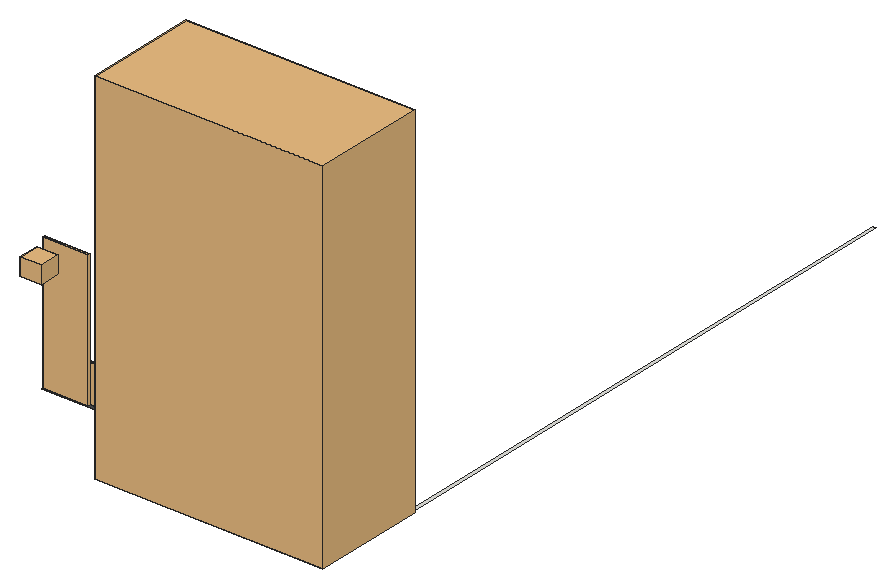
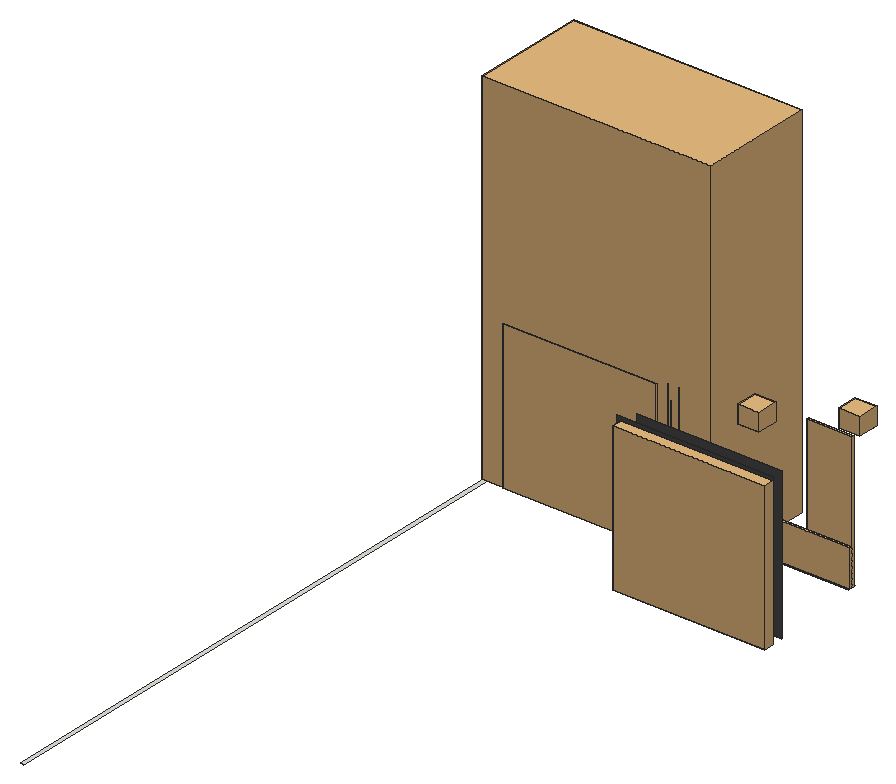
# SketchUp Ruby script. Lengths in inches.
U = 1.inch
M = Sketchup.active_model
def pt(a) = Geom::Point3d.new(a.map { |v| v * U })
def face(e, loops, mat)
  f = e.add_face(loops[0].map { |a| pt(a) })
  loops[1..].each { |l| e.add_face(l.map { |a| pt(a) }).erase! }
  f.material = f.back_material = mat if mat
  f
end
# faces: each face lists its corners as indices into pts; further lists are holes
def faces(e, pts, list, mat = nil) = list.each { |f| face(e, (f[0].is_a?(Array) ? f : [f]).map { |l| l.map { |i| pts[i] } }, mat) }
# xy, xz, yz: faces in a plane at the given z, y or x. An outline is a flat list of corners, or four numbers for a rectangle; further outlines are holes
def ring(l) = l.size == 4 ? [[l[0], l[1]], [l[2], l[1]], [l[2], l[3]], [l[0], l[3]]] : l.each_slice(2).to_a
def flat(e, list, mat, &to3) = list.each { |f| face(e, (f[0].is_a?(Array) ? f : [f]).map { |l| ring(l).map { |u, v| to3.(u, v) } }, mat) }
def xy(e, z, list, mat = nil) = flat(e, list, mat) { |x, y| [x, y, z] }
def xz(e, y, list, mat = nil) = flat(e, list, mat) { |x, z| [x, y, z] }
def yz(e, x, list, mat = nil) = flat(e, list, mat) { |y, z| [x, y, z] }
def lines(e, pts, list) = list.each { |a, b| e.add_line(pt(pts[a]), pt(pts[b])) }
# prism: a flat outline (further loops are holes) pulled along v
def prism(e, loops, v, mat = nil)
  f = face(e, loops, mat); d = Geom::Vector3d.new(v.map { |x| x * U })
  f.pushpull(f.normal.samedirection?(d) ? d.length : -d.length)
end
def box(e, o, s, mat = nil) = prism(e, [[o, [o[0] + s[0], o[1], o[2]], [o[0] + s[0], o[1] + s[1], o[2]], [o[0], o[1] + s[1], o[2]]]], [0, 0, s[2]], mat)
def at(x, y, z, deg = 0) = Geom::Transformation.translation(pt([x, y, z])) * Geom::Transformation.rotation(ORIGIN, Z_AXIS, deg.degrees)
def axes(o, x, y, z) = Geom::Transformation.new([*x, 0, *y, 0, *z, 0, *pt(o).to_a, 1])
def part(name) = M.definitions.add(name)
# library, detail: a bought-in or finely detailed component or shape, given as its bounding box
def library(name, o, s) = part(name).tap { |d| box(d.entities, o, s) }
def detail(e, o, s) = box(e.add_group.entities, o, s)
def put(e, d, t, mat = nil) = e.add_instance(d, t).tap { |i| i.material = mat if mat }
def group(e, t, mat = nil) = e.add_group.tap { |g| g.transformation = t; g.material = mat if mat }.entities
root = M.entities
M.materials.add("1423 AP 8230 BENTONITE").color = [77, 75, 77]
M.materials.add("1427 AP 686 ARMOUR-N").color = [184, 186, 189]
M.materials.add("[Wood Cherry Original]").color = [100, 65, 42]
M.materials.add("[Wood Veneer 01]").color = [99, 65, 43]
c1 = library("Curtains",[0,0,0],[121.73,8.19,117.22])
c2 = library("Group\#13",[-25,-1,0],[182,91,288])
c3 = library("Untitled",[0,0,0],[96,5.09,80])
c4 = library("Group\#19",[0,-2,0],[36,2,114])
c5 = library("Group\#35",[-36,0,0],[116,2,29.75])
c6 = library("2",[-6.43,-6.43,-13.78],[16.84,16.84,13.78])
xy(root,126,[[287,192,290,672]])
xy(root,126,[[151.78,192,151.57,192.01,151.35,192.01,150.91,192.03,150.7,192.05,150.48,192.0625,150.26,192.08,150.05,192.11,149.83,192.13,149.61,192.16,149.4,192.1875,149.18,192.22,148.97,192.26,148.76,192.29,148.54,192.34,148.12,192.42,147.9,192.47,147.69,192.52,147.48,192.58,147.27,192.63,147.0625,192.69,146.85,192.75,146.64,192.82,146.4375,192.88,146.23,192.95,146.03,193.02,145.82,193.09,145.62,193.17,145.41,193.25,145.01,193.41,144.8125,193.5,144.61,193.59,144.41,193.68,144.22,193.77,144.02,193.86,143.83,193.96,143.63,194.0625,143.44,194.16,143.25,194.27,142.875,194.48,142.6875,194.6,142.5,194.71,142.32,194.83,142.14,194.94,141.95,195.0625,141.77,195.1875,141.6,195.3125,141.42,195.4375,141.24,195.57,140.9,195.83,140.73,195.97,140.56,196.1,140.39,196.24,140.23,196.38,140.0625,196.53,139.9,196.67,139.58,196.97,139.43,197.12,139.27,197.27,139.12,197.43,138.97,197.58,138.67,197.9,138.53,198.0625,138.38,198.23,138.24,198.39,138.1,198.56,137.97,198.73,137.83,198.9,137.57,199.24,137.4375,199.42,137.3125,199.6,137.1875,199.77,137.0625,199.95,136.94,200.14,136.83,200.32,136.71,200.5,136.6,200.6875,136.48,200.875,136.27,201.25,136.16,201.44,136.0625,201.63,135.96,201.83,135.86,202.02,135.77,202.22,135.68,202.41,135.59,202.61,135.5,202.8125,135.41,203.01,135.25,203.41,135.17,203.62,135.09,203.82,135.02,204.03,134.95,204.23,134.88,204.4375,134.82,204.64,134.75,204.85,134.69,205.0625,134.63,205.27,134.58,205.48,134.52,205.69,134.47,205.9,134.42,206.12,134.34,206.54,134.29,206.76,134.26,206.97,134.22,207.18,134.1875,207.4,134.16,207.61,134.13,207.83,134.11,208.05,134.08,208.26,134.0625,208.48,134.05,208.7,134.03,208.91,134.01,209.35,134.01,209.57,134,209.78,134,252,128,252,128,261,143,261,143,209.78,143.01,209.67,143.01,209.57,143.02,209.46,143.02,209.35,143.05,209.02,143.07,208.92,143.09,208.7,143.13,208.48,143.15,208.38,143.17,208.27,143.1875,208.16,143.21,208.06,143.24,207.95,143.26,207.85,143.29,207.74,143.32,207.64,143.35,207.53,143.375,207.43,143.41,207.32,143.47,207.12,143.51,207.01,143.55,206.91,143.58,206.81,143.625,206.71,143.66,206.61,143.71,206.51,143.79,206.31,143.84,206.21,143.88,206.11,143.98,205.91,144.03,205.82,144.08,205.72,144.13,205.625,144.1875,205.53,144.24,205.4375,144.3,205.34,144.35,205.25,144.59,204.89,144.66,204.8,144.78,204.62,144.85,204.54,144.92,204.45,144.98,204.36,145.12,204.2,145.19,204.11,145.26,204.03,145.34,203.95,145.48,203.79,145.56,203.71,145.64,203.64,145.71,203.56,145.79,203.48,145.95,203.34,146.03,203.26,146.11,203.19,146.2,203.12,146.36,202.98,146.45,202.92,146.54,202.85,146.62,202.78,146.8,202.66,146.89,202.59,147.25,202.35,147.34,202.3,147.4375,202.24,147.53,202.1875,147.625,202.13,147.72,202.08,147.82,202.03,147.91,201.98,148.11,201.88,148.21,201.84,148.31,201.79,148.51,201.71,148.61,201.66,148.71,201.625,148.81,201.58,148.91,201.55,149.01,201.51,149.12,201.47,149.32,201.41,149.43,201.375,149.53,201.35,149.64,201.32,149.74,201.29,149.85,201.26,149.95,201.24,150.06,201.21,150.16,201.1875,150.27,201.17,150.38,201.15,150.48,201.13,150.7,201.09,150.92,201.07,151.02,201.05,151.35,201.02,151.46,201.02,151.57,201.01,151.67,201.01,151.78,201,170,201,170,192]],"1423 AP 8230 BENTONITE")
xy(root,132,[[18,180,134,186]],"1423 AP 8230 BENTONITE")
xy(root,216,[[56,252,128,261]],"1423 AP 8230 BENTONITE")
xy(root,222,[[170,192,254,201]],"1423 AP 8230 BENTONITE")
xz(root,201,[[151.78,126,151.89,246],[151.89,126,151.89,246,281,246,281,126,254,126,254,222,170,222,170,126]],"1423 AP 8230 BENTONITE")
xz(root,201.01,[[151.57,126,151.67,246]],"1423 AP 8230 BENTONITE")
xz(root,201.02,[[151.35,126,151.46,246]],"1423 AP 8230 BENTONITE")
xz(root,252,[[18,126,56,126,56,216,128,216,128,126,134,126,134,246,18,246]],"1423 AP 8230 BENTONITE")
xz(root,261,[[18,126,18,246,143,246,143,126,128,126,128,216,56,216,56,126]],"1423 AP 8230 BENTONITE")
yz(root,56,[[252,126,261,216]],"1423 AP 8230 BENTONITE")
yz(root,128,[[252,126,261,216]],"1423 AP 8230 BENTONITE")
yz(root,134,[[209.78,126,210,246]],"1423 AP 8230 BENTONITE")
yz(root,134.01,[[209.35,126,209.57,246]],"1423 AP 8230 BENTONITE")
yz(root,143,[[209.78,126,209.89,246]],"1423 AP 8230 BENTONITE")
yz(root,143.01,[[209.57,126,209.67,246]],"1423 AP 8230 BENTONITE")
yz(root,143.02,[[209.35,126,209.46,246]],"1423 AP 8230 BENTONITE")
p = [[151.02,201.05,246],[151.13,201.04,246],[151.13,201.04,126],[151.02,201.05,126],[151.24,201.03,246],[151.24,201.03,126],
  [151.35,201.02,246],[151.35,201.02,126],[151.46,201.02,246],[151.57,201.01,246],[151.57,201.01,126],[151.46,201.02,126],
  [151.67,201.01,246],[151.78,201,246],[151.78,201,126],[151.67,201.01,126],[150.27,201.17,246],[150.38,201.15,246],
  [150.38,201.15,126],[150.27,201.17,126],[150.48,201.13,246],[150.48,201.13,126],[150.59,201.11,246],[150.59,201.11,126],
  [150.7,201.09,246],[150.7,201.09,126],[150.81,201.08,246],[150.81,201.08,126],[150.92,201.07,246],[150.92,201.07,126],
  [149.85,201.26,246],[149.95,201.24,246],[149.95,201.24,126],[149.85,201.26,126],[150.06,201.21,246],[150.06,201.21,126],
  [150.16,201.1875,246],[150.16,201.1875,126],[149.43,201.375,246],[149.53,201.35,246],[149.53,201.35,126],[149.43,201.375,126],
  [149.64,201.32,246],[149.64,201.32,126],[149.74,201.29,246],[149.74,201.29,126],[149.12,201.47,246],[149.22,201.44,246],
  [149.22,201.44,126],[149.12,201.47,126],[149.32,201.41,246],[149.32,201.41,126],[148.81,201.58,246],[148.91,201.55,246],
  [148.91,201.55,126],[148.81,201.58,126],[149.01,201.51,246],[149.01,201.51,126],[148.61,201.66,246],[148.71,201.625,246],
  [148.71,201.625,126],[148.61,201.66,126],[148.31,201.79,246],[148.41,201.75,246],[148.41,201.75,126],[148.31,201.79,126],
  [148.51,201.71,246],[148.51,201.71,126],[148.11,201.88,246],[148.21,201.84,246],[148.21,201.84,126],[148.11,201.88,126],
  [147.91,201.98,246],[148.01,201.93,246],[148.01,201.93,126],[147.91,201.98,126],[147.72,202.08,246],[147.82,202.03,246],
  [147.82,202.03,126],[147.72,202.08,126],[147.53,202.1875,246],[147.625,202.13,246],[147.625,202.13,126],[147.53,202.1875,126],
  [147.34,202.3,246],[147.4375,202.24,246],[147.4375,202.24,126],[147.34,202.3,126],[147.25,202.35,246],[147.25,202.35,126],
  [147.07,202.47,246],[147.16,202.41,246],[147.16,202.41,126],[147.07,202.47,126],[146.89,202.59,246],[146.98,202.53,246],
  [146.98,202.53,126],[146.89,202.59,126],[146.8,202.66,246],[146.8,202.66,126],[146.62,202.78,246],[146.71,202.72,246],
  [146.71,202.72,126],[146.62,202.78,126],[146.45,202.92,246],[146.54,202.85,246],[146.54,202.85,126],[146.45,202.92,126],
  [146.36,202.98,246],[146.36,202.98,126],[146.28,203.05,246],[146.28,203.05,126],[146.11,203.19,246],[146.2,203.12,246],
  [146.2,203.12,126],[146.11,203.19,126],[146.03,203.26,246],[146.03,203.26,126],[145.87,203.41,246],[145.95,203.34,246],
  [145.95,203.34,126],[145.87,203.41,126],[145.79,203.48,246],[145.79,203.48,126],[145.71,203.56,246],[145.71,203.56,126],
  [145.64,203.64,246],[145.64,203.64,126],[145.56,203.71,246],[145.56,203.71,126],[145.48,203.79,246],[145.48,203.79,126],
  [145.41,203.87,246],[145.41,203.87,126],[145.34,203.95,246],[145.34,203.95,126],[145.19,204.11,246],[145.26,204.03,246],
  [145.26,204.03,126],[145.19,204.11,126],[145.12,204.2,246],[145.12,204.2,126],[145.05,204.28,246],[145.05,204.28,126],
  [144.98,204.36,246],[144.98,204.36,126],[144.85,204.54,246],[144.92,204.45,246],[144.92,204.45,126],[144.85,204.54,126],
  [144.78,204.62,246],[144.78,204.62,126],[144.72,204.71,246],[144.72,204.71,126],[144.66,204.8,246],[144.66,204.8,126],
  [144.59,204.89,246],[144.59,204.89,126],[144.53,204.98,246],[144.53,204.98,126],[144.47,205.07,246],[144.47,205.07,126],
  [144.41,205.16,246],[144.41,205.16,126],[144.35,205.25,246],[144.35,205.25,126],[144.24,205.4375,246],[144.3,205.34,246],
  [144.3,205.34,126],[144.24,205.4375,126],[144.1875,205.53,246],[144.1875,205.53,126],[144.13,205.625,246],[144.13,205.625,126],
  [144.08,205.72,246],[144.08,205.72,126],[144.03,205.82,246],[144.03,205.82,126],[143.98,205.91,246],[143.98,205.91,126],
  [143.93,206.01,246],[143.93,206.01,126],[143.88,206.11,246],[143.88,206.11,126],[143.84,206.21,246],[143.84,206.21,126],
  [143.79,206.31,246],[143.79,206.31,126],[143.75,206.41,246],[143.75,206.41,126],[143.71,206.51,246],[143.71,206.51,126],
  [143.66,206.61,246],[143.66,206.61,126],[143.625,206.71,246],[143.625,206.71,126],[143.58,206.81,246],[143.58,206.81,126],
  [143.55,206.91,246],[143.55,206.91,126],[143.51,207.01,246],[143.51,207.01,126],[143.47,207.12,246],[143.47,207.12,126],
  [143.44,207.22,246],[143.44,207.22,126],[143.41,207.32,246],[143.41,207.32,126],[143.375,207.43,246],[143.375,207.43,126],
  [143.35,207.53,246],[143.35,207.53,126],[143.32,207.64,246],[143.32,207.64,126],[143.29,207.74,246],[143.29,207.74,126],
  [143.26,207.85,246],[143.26,207.85,126],[143.24,207.95,246],[143.24,207.95,126],[143.21,208.06,246],[143.21,208.06,126],
  [143.1875,208.16,246],[143.1875,208.16,126],[143.17,208.27,246],[143.17,208.27,126],[143.15,208.38,246],[143.15,208.38,126],
  [143.13,208.48,246],[143.13,208.48,126],[143.11,208.59,246],[143.11,208.59,126],[143.09,208.7,246],[143.09,208.7,126],
  [134.05,208.7,246],[134.03,208.91,246],[134.03,208.91,126],[134.05,208.7,126],[143.08,208.81,246],[143.08,208.81,126],
  [143.07,208.92,246],[143.07,208.92,126],[134.02,209.13,246],[134.02,209.13,126],[143.05,209.02,246],[143.05,209.02,126],
  [143.04,209.13,246],[143.04,209.13,126],[134.01,209.35,246],[134.01,209.35,126],[143.03,209.24,246],[143.03,209.24,126],
  [143.02,209.35,246],[143.02,209.35,126],[143.01,209.57,246],[143.02,209.46,246],[143.02,209.46,126],[143.01,209.57,126],
  [134.01,209.57,246],[134,209.78,246],[134,209.78,126],[134.01,209.57,126],[143,209.78,246],[143.01,209.67,246],
  [143.01,209.67,126],[143,209.78,126]]
faces(root,p,[[0,1,2,3],[1,4,5,2],[4,6,7,5],[8,9,10,11],[12,13,14,15],[16,17,18,19],[17,20,21,18],[20,22,23,21],
  [22,24,25,23],[24,26,27,25],[26,28,29,27],[28,0,3,29],[30,31,32,33],[31,34,35,32],[34,36,37,35],[36,16,19,37],
  [38,39,40,41],[39,42,43,40],[42,44,45,43],[44,30,33,45],[46,47,48,49],[47,50,51,48],[50,38,41,51],[52,53,54,55],
  [53,56,57,54],[56,46,49,57],[58,59,60,61],[59,52,55,60],[62,63,64,65],[63,66,67,64],[66,58,61,67],[68,69,70,71],
  [69,62,65,70],[72,73,74,75],[73,68,71,74],[76,77,78,79],[77,72,75,78],[80,81,82,83],[81,76,79,82],[84,85,86,87],
  [85,80,83,86],[88,84,87,89],[90,91,92,93],[91,88,89,92],[94,95,96,97],[95,90,93,96],[98,94,97,99],[100,101,102,103],
  [101,98,99,102],[104,105,106,107],[105,100,103,106],[108,104,107,109],[110,108,109,111],[112,113,114,115],[113,110,111,114],[116,112,115,117],
  [118,119,120,121],[119,116,117,120],[122,118,121,123],[124,122,123,125],[126,124,125,127],[128,126,127,129],[130,128,129,131],[132,130,131,133],
  [134,132,133,135],[136,137,138,139],[137,134,135,138],[140,136,139,141],[142,140,141,143],[144,142,143,145],[146,147,148,149],[147,144,145,148],
  [150,146,149,151],[152,150,151,153],[154,152,153,155],[156,154,155,157],[158,156,157,159],[160,158,159,161],[162,160,161,163],[164,162,163,165],
  [166,167,168,169],[167,164,165,168],[170,166,169,171],[172,170,171,173],[174,172,173,175],[176,174,175,177],[178,176,177,179],[180,178,179,181],
  [182,180,181,183],[184,182,183,185],[186,184,185,187],[188,186,187,189],[190,188,189,191],[192,190,191,193],[194,192,193,195],[196,194,195,197],
  [198,196,197,199],[200,198,199,201],[202,200,201,203],[204,202,203,205],[206,204,205,207],[208,206,207,209],[210,208,209,211],[212,210,211,213],
  [214,212,213,215],[216,214,215,217],[218,216,217,219],[220,218,219,221],[222,220,221,223],[224,222,223,225],[226,224,225,227],[228,226,227,229],
  [230,228,229,231],[232,230,231,233],[234,235,236,237],[238,232,233,239],[240,238,239,241],[235,242,243,236],[244,240,241,245],[246,244,245,247],
  [242,248,249,243],[250,246,247,251],[252,250,251,253],[254,255,256,257],[258,259,260,261],[262,263,264,265]],"1423 AP 8230 BENTONITE")
put(root,c1,at(151.89,202.72,126),"1423 AP 8230 BENTONITE")
put(root,c1,at(18,261,126),"1423 AP 8230 BENTONITE")
put(root,c2,at(134,120,126),"1427 AP 686 ARMOUR-N")
put(root,c3,axes([56,254,126],[0.75,0,0],[0,1,0],[0,0,1.125]),"1423 AP 8230 BENTONITE")
put(root,c4,axes([233,134,126],[1,0,0],[0,1,0],[0,0,2.10526]),"[Wood Cherry Original]")
put(root,c5,at(54,183,132),"[Wood Veneer 01]")
put(root,c4,axes([18,182.5,132],[1,0,0],[0,1,0],[0,0,0.94737]),"[Wood Cherry Original]")
put(root,c6,at(33.01,153.93,243.38))
put(root,c6,at(85.01,189.01,243.38))
put(root,c6,at(137.01,153.93,243.38))
